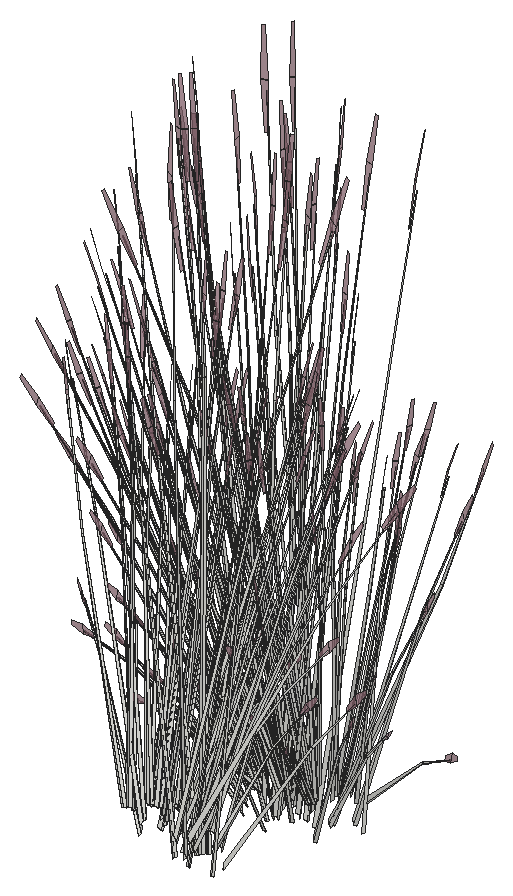
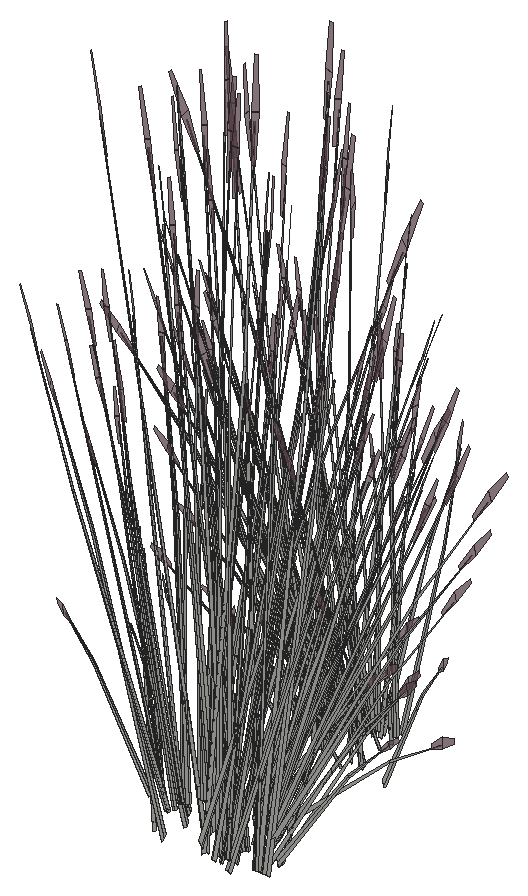
# SketchUp Ruby script. Lengths in inches.
U = 1.inch
M = Sketchup.active_model
def pt(a) = Geom::Point3d.new(a.map { |v| v * U })
def face(e, loops, mat)
  f = e.add_face(loops[0].map { |a| pt(a) })
  loops[1..].each { |l| e.add_face(l.map { |a| pt(a) }).erase! }
  f.material = f.back_material = mat if mat
  f
end
# faces: each face lists its corners as indices into pts; further lists are holes
def faces(e, pts, list, mat = nil) = list.each { |f| face(e, (f[0].is_a?(Array) ? f : [f]).map { |l| l.map { |i| pts[i] } }, mat) }
# xy, xz, yz: faces in a plane at the given z, y or x. An outline is a flat list of corners, or four numbers for a rectangle; further outlines are holes
def ring(l) = l.size == 4 ? [[l[0], l[1]], [l[2], l[1]], [l[2], l[3]], [l[0], l[3]]] : l.each_slice(2).to_a
def flat(e, list, mat, &to3) = list.each { |f| face(e, (f[0].is_a?(Array) ? f : [f]).map { |l| ring(l).map { |u, v| to3.(u, v) } }, mat) }
def xy(e, z, list, mat = nil) = flat(e, list, mat) { |x, y| [x, y, z] }
def xz(e, y, list, mat = nil) = flat(e, list, mat) { |x, z| [x, y, z] }
def yz(e, x, list, mat = nil) = flat(e, list, mat) { |y, z| [x, y, z] }
def lines(e, pts, list) = list.each { |a, b| e.add_line(pt(pts[a]), pt(pts[b])) }
# prism: a flat outline (further loops are holes) pulled along v
def prism(e, loops, v, mat = nil)
  f = face(e, loops, mat); d = Geom::Vector3d.new(v.map { |x| x * U })
  f.pushpull(f.normal.samedirection?(d) ? d.length : -d.length)
end
def box(e, o, s, mat = nil) = prism(e, [[o, [o[0] + s[0], o[1], o[2]], [o[0] + s[0], o[1] + s[1], o[2]], [o[0], o[1] + s[1], o[2]]]], [0, 0, s[2]], mat)
def at(x, y, z, deg = 0) = Geom::Transformation.translation(pt([x, y, z])) * Geom::Transformation.rotation(ORIGIN, Z_AXIS, deg.degrees)
def axes(o, x, y, z) = Geom::Transformation.new([*x, 0, *y, 0, *z, 0, *pt(o).to_a, 1])
def part(name) = M.definitions.add(name)
# library, detail: a bought-in or finely detailed component or shape, given as its bounding box
def library(name, o, s) = part(name).tap { |d| box(d.entities, o, s) }
def detail(e, o, s) = box(e.add_group.entities, o, s)
def put(e, d, t, mat = nil) = e.add_instance(d, t).tap { |i| i.material = mat if mat }
def group(e, t, mat = nil) = e.add_group.tap { |g| g.transformation = t; g.material = mat if mat }.entities
root = M.entities
M.materials.add("LightPink_Translucent").color = [144, 107, 117]
M.materials["LightPink_Translucent"].alpha = 0.75
c1 = part("blade")
p = [[2.15,0.21,22],[0,0.17,0],[0.09,0.45,0],[2.18,0.31,22],[2.29,0.31,22],[0.38,0.45,0],
  [2.48,0.24,33],[2.49,0.24,33],[2.48,0.22,33]]
faces(c1.entities,p,[[0,1,2,3],[4,5,2,3],[6,3,4,7],[8,0,3,6]])
c2 = part("seeds")
p = [[0.3,-0.1,1.38],[-0.01,-0.03,1.59],[-0.01,-0.03,0.03],[0.14,-0.07,-0.07],[0.29,-0.03,3],[0.15,0.01,3.11]]
faces(c2.entities,p,[[0,1,2,3],[1,0,4,5]],"LightPink_Translucent")
c3 = part("blade with seeds")
put(c3.entities,c1,at(0,0,0))
put(c3.entities,c2,axes([2.4,0.25,30.99],[1.5799,-0.05474,1.17369],[-0.12525,1.92788,0.29478],[-0.07173,-0.02425,1.56792]))
put(root,c3,axes([340.3,184.53,6.82],[-0.77872,0.09325,-0.35414],[-0.20563,-0.53305,0.4572],[-0.22316,0.14318,0.87481]))
put(root,c3,axes([347.67,185.27,7.03],[-0.65964,0.42992,0.48003],[-0.5689,-0.45657,0.3958],[0.30948,0.0793,0.9933]))
put(root,c3,axes([339.17,185.73,7.9375],[0.78943,0.17416,-0.06488],[-0.24284,0.53604,-0.29416],[-0.12912,0.08139,0.97024]))
put(root,c3,axes([344.77,184.74,4.35],[-0.60257,0.49041,-0.62353],[-0.74854,-0.44469,-0.16365],[-0.24146,0.12234,1.37633]))
put(root,c3,axes([345.57,185.76,7.34],[-0.13817,-0.52554,0.35414],[0.78985,-0.13877,-0.4572],[0.21215,0.1506,0.87481]))
put(root,c3,axes([345.84,185.57,4.625],[1.11998,0.21207,0.30756],[-0.2802,0.75803,-0.36492],[-0.18537,0.09487,1.64885]))
put(root,c3,axes([345.76,186.08,4.3125],[-0.83726,0.32623,-0.49651],[-0.50045,-0.58498,0],[-0.19069,0.0743,1.57504]))
put(root,c3,axes([348.54,184.15,4.3125],[0,0.65246,-0.49651],[-1.00089,0,0],[0,0.1486,1.57504]))
put(root,c3,axes([346.04,184.22,6.17],[-0.3323,-0.11241,1.71376],[0.68769,-0.4716,0.13857],[0.42861,0.21275,0.73262]))
put(root,c3,axes([346.1,182.74,6.77],[-0.77304,-0.33901,1.38283],[0.81626,-0.52782,0.59665],[0.24941,0.31809,1.33663]))
put(root,c3,axes([340.53,184.17,7.33],[0.82753,0.35977,-0.1216],[-0.47675,0.52101,-0.67495],[-0.2338,0.18111,1.02557]))
put(root,c3,axes([347.27,185.5,5.06],[-0.5037,-0.18761,1.1486],[0.6504,-0.19062,0.84392],[0.17543,0.16147,0.25299]))
put(root,c3,axes([345.5,186.04,7.33],[0.53309,-0.55848,-0.1216],[0.77201,0.32175,-0.67495],[0.26836,0.15779,1.02557]))
put(root,c3,axes([341.64,184.01,6.17],[0.22344,-0.20048,1.71376],[0.56419,0.54113,0.13857],[-0.38697,0.24643,0.73262]))
put(root,c3,axes([340.94,184.6,6.97],[0.22982,0.59576,-0.51099],[-0.87033,0.10422,-0.3958],[-0.24941,0.16002,0.97773]))
put(root,c3,axes([341.98,185.28,7.34],[0.60531,-0.34352,0.35414],[0.573,0.39225,-0.4572],[-0.08718,0.19929,0.87481]))
put(root,c3,axes([346.52,185.98,4.67],[0.55932,0.6538,0],[-0.93577,0.36461,-0.51607],[-0.21313,0.08304,1.63711]))
put(root,c3,axes([344.8,186.5,7],[0.00265,-0.07899,1.77383],[0.76665,-0.34851,-0.16761],[0.2663,0.12439,0.31391]))
put(root,c3,axes([347.41,186.2,3.79],[0.06518,-0.0942,1.76342],[0.82057,-0.27742,-0.26939],[0.24877,0.14358,0.30037]))
put(root,c3,axes([346.04,183.39,5.13],[-0.02444,-0.61432,1.41272],[1.10603,0.15924,0.59816],[-0.26159,0.33615,1.3335]))
put(root,c3,axes([346.33,184.06,4.39],[0.32803,0.59738,-0.69212],[-0.94492,0.21515,-0.18165],[0.03626,0.20229,1.52773]))
put(root,c3,axes([341.4375,185.59,7.02],[-0.73517,-0.0304,0.0643],[0.02016,-0.45906,0.50621],[-0.07693,0.17585,0.77189]))
put(root,c3,axes([339.875,186.12,3.79],[0.12,0.06519,1.76342],[0.20347,0.60397,-0.26939],[-0.26596,0.12879,0.30037]))
put(root,c3,axes([341.67,185.63,7.03],[-0.63704,-0.44518,0.48003],[0.67652,-0.38394,0.3958],[-0.11751,0.20886,0.9933]))
put(root,c3,axes([346.13,185.76,6.97],[0.88277,-0.1551,-0.51099],[0.15442,0.58737,-0.3958],[0.23711,0.16832,0.97773]))
put(root,c3,axes([343.68,185.85,7.34],[0.2697,-0.50175,0.35414],[0.78684,0.14635,-0.4572],[0.07215,0.20201,0.87481]))
put(root,c3,axes([347.35,186.35,4.96],[-0.57368,-0.02046,1.0506],[0.37886,-0.43461,0.58006],[0.22663,0.15441,0.8241]))
put(root,c3,axes([345.7,186.24,7.02],[-0.4066,0.41448,0.0643],[-0.57901,-0.24131,0.50621],[0.18719,0.13288,0.77189]))
put(root,c3,axes([344.74,187.64,7.9375],[0.61821,-0.37431,-0.06488],[0.56645,0.40995,-0.29416],[0.03988,0.11616,0.97024]))
put(root,c3,axes([345.87,186.125,7.03],[-0.88979,0.14973,0.48003],[-0.15442,-0.58737,0.3958],[0.20926,0.17311,0.9933]))
put(root,c3,axes([341.48,184.5,6.17],[0.16657,-0.22426,1.71376],[0.69879,0.4641,0.13857],[-0.31524,0.28926,0.73262]))
put(root,c3,axes([345.48,185.3,4.88],[0.01579,-0.21629,1.43002],[0.75442,-0.24159,-0.30754],[0.23289,0.25887,0.61141]))
put(root,c3,axes([343.4375,186.3,7.02],[-0.6592,0.22175,0.0643],[-0.32265,-0.40436,0.50621],[0.06366,0.17825,0.77189]))
put(root,c3,axes([341.67,185.77,6.82],[-0.60531,0.34352,-0.35414],[-0.573,-0.39225,0.4572],[-0.08718,0.19929,0.87481]))
put(root,c3,axes([339.58,185.67,7.01],[-0.02224,0.12912,1.74944],[0.63107,0.44917,-0.27667],[-0.16521,0.21241,0.14031]))
put(root,c3,axes([341.6,185.375,7.69],[0.98321,0.03233,-0.13498],[-0.02687,0.61208,-0.74919],[-0.0683,0.23574,1.13838]))
put(root,c3,axes([343.42,186.06,7.33],[0.87543,-0.30377,-0.1216],[0.4302,0.53915,-0.67495],[0.1155,0.2272,1.02557]))
put(root,c3,axes([343.67,186.26,7.36],[-0.88151,-0.17057,0.53283],[0.30143,-0.56078,0.43934],[0.05297,0.22053,1.10256]))
put(root,c3,axes([342.05,187.1,5.06],[-0.02315,-0.38796,1.1486],[0.57853,0.27671,0.84392],[-0.11378,0.18492,0.25299]))
put(root,c3,axes([343.58,186.18,3.79],[0.14478,-0.0355,1.76342],[0.8709,0.19542,-0.26939],[0.02547,0.22025,0.30037]))
put(root,c3,axes([342.27,185.61,7.3],[0.64041,0.4384,-0.5672],[-0.67652,0.38394,-0.43934],[-0.09744,0.22274,1.08528]))
put(root,c3,axes([341.57,186.26,5.12],[0.8127,-0.11554,0.06507],[0.18684,0.46549,-0.86304],[-0.05152,0.23564,0.7736]))
put(root,c3,axes([344.17,186.03,6.97],[0.87941,0.16356,-0.51099],[-0.30143,0.56078,-0.3958],[0.08064,0.22578,0.97773]))
put(root,c3,axes([344.67,184.875,6.17],[-0.2045,-0.20949,1.71376],[0.94495,-0.17636,0.13857],[0.21357,0.32887,0.73262]))
put(root,c3,axes([343.77,186.375,6.82],[-0.2697,0.50175,-0.35414],[-0.78684,-0.14635,0.4572],[0.07215,0.20201,0.87481]))
put(root,c3,axes([342.42,196.51,3.875],[0.2045,0.20949,1.71376],[-0.94495,0.17636,0.13857],[-0.21357,-0.32887,0.73262]))
put(root,c3,axes([342.07,185.41,7.63],[-0.02328,0.60353,-0.7886],[-0.98022,-0.04053,0.09517],[-0.10344,0.25568,1.11556]))
put(root,c3,axes([339.51,186.99,7],[0.10149,-0.03939,1.77383],[0.83886,0.26202,-0.16761],[-0.01971,0.21816,0.31391]))
put(root,c3,axes([343.98,195.12,4.72],[-0.13683,-0.09148,1.74944],[-0.91315,0.058,-0.27667],[-0.14574,-0.2188,0.14031]))
put(root,c3,axes([343,184.98,6.17],[-0.0219,-0.25042,1.71376],[0.94901,0.16613,0.13857],[-0.0587,0.35688,0.73262]))
put(root,c3,axes([346.1,196.2,2.59],[-0.25429,0.13207,1.43002],[-0.76157,-0.23115,-0.30754],[0.14117,-0.28747,0.61141]))
put(root,c3,axes([344.94,196.66,4.98],[-0.42698,-0.53052,-0.71045],[0.87893,-0.29566,0.08574],[-0.09984,-0.25633,1.00501]))
put(root,c3,axes([342.16,195.95,2.59],[-0.05417,0.21344,1.43002],[-0.79196,0.17867,-0.30754],[-0.18512,-0.27588,0.61141]))
put(root,c3,axes([343.85,185.92,7.27],[0.42698,0.53052,-0.71045],[-0.87893,0.29566,0.08574],[0.09984,0.25633,1.00501]))
put(root,c3,axes([344.2,195.49,1.49],[-0.15005,0.02351,1.76342],[-0.82981,-0.26461,-0.26939],[0.01392,-0.22072,0.30037]))
put(root,c3,axes([341.38,186.76,4.88],[0.28231,-0.10293,1.43002],[0.69701,0.31035,-0.30754],[-0.20746,0.26854,0.61141]))
put(root,c3,axes([343.21,187.26,7.01],[0.1134,0.10507,1.74944],[0.91515,0.04128,-0.27667],[0.09203,0.23172,0.14031]))
put(root,c3,axes([346.72,197.18,4.98],[0.02328,-0.60353,-0.71045],[0.98022,0.04053,0.08574],[0.10344,-0.25568,1.00501]))
put(root,c3,axes([348.09,196.24,4.72],[-0.00864,-0.12985,1.74944],[-0.72937,-0.3753,-0.27667],[0.11277,-0.2275,0.14031]))
put(root,c3,axes([345.02,196.21,4.53],[0.2697,-0.50175,-0.35414],[0.78684,0.14635,0.4572],[-0.07215,-0.20201,0.87481]))
put(root,c3,axes([345.62,196.875,3.875],[-0.16657,0.22426,1.71376],[-0.69879,-0.4641,0.13857],[0.31524,-0.28926,0.73262]))
put(root,c3,axes([347.89,195.77,4.71],[-0.09085,0.04984,1.77383],[-0.89014,-0.16814,-0.16761],[-0.03222,-0.21748,0.31391]))
put(root,c3,axes([344.62,196.56,4.68],[-0.87941,-0.16356,-0.51099],[0.30143,-0.56078,-0.3958],[-0.08064,-0.22578,0.97773]))
put(root,c3,axes([345.16,195.15,2.77],[0.11476,0.38047,1.1486],[-0.63664,-0.21072,0.84392],[0.06851,-0.19481,0.25299]))
put(root,c3,axes([346.52,196.98,4.68],[-0.64041,-0.4384,-0.51099],[0.67652,-0.38394,-0.3958],[0.09744,-0.22274,0.97773]))
put(root,c3,axes([341.74,186.26,5.66],[0.01966,-0.33682,1.54345],[0.88405,0.17791,0.21329],[-0.0766,0.35897,0.72882]))
put(root,c3,axes([343.05,194.82,4.71],[-0.01669,0.07821,1.77383],[-0.82314,0.28383,-0.16761],[-0.24223,-0.14508,0.31391]))
put(root,c3,axes([342.87,196.21,5.09],[0.99656,-0.1677,0.53763],[0.17295,0.65785,0.4433],[-0.23438,-0.19388,1.11249]))
put(root,c3,axes([345.12,196.33,4.73],[0.88151,0.17057,0.48003],[-0.30143,0.56078,0.3958],[-0.05297,-0.22053,0.9933]))
put(root,c3,axes([345.37,196.53,5.03],[-0.87543,0.30377,-0.1216],[-0.4302,-0.53915,-0.67495],[-0.1155,-0.2272,1.02557]))
put(root,c3,axes([347.19,197.21,5.03],[-0.98321,-0.03233,-0.1216],[0.02687,-0.61208,-0.67495],[0.0683,-0.23574,1.02557]))
put(root,c3,axes([347.12,196.82,4.53],[0.60531,-0.34352,-0.35414],[0.573,0.39225,0.4572],[0.08718,-0.19929,0.87481]))
put(root,c3,axes([341.89,195.61,2.77],[0.46666,0.22709,1.1486],[-0.67962,0.13651,0.84392],[-0.14541,-0.17452,0.25299]))
put(root,c3,axes([345.35,196.29,4.73],[0.6592,-0.22175,0.0643],[0.32265,0.40436,0.50621],[-0.06366,-0.17825,0.77189]))
put(root,c3,axes([343.02,196.8125,4.98],[-0.76283,-0.31537,-0.71045],[0.54213,-0.55263,0.08574],[-0.27638,-0.1883,1.00501]))
put(root,c3,axes([342.75,196.4,4.53],[-0.13817,-0.52554,-0.35414],[0.78985,-0.13877,0.4572],[-0.21215,-0.1506,0.87481]))
put(root,c3,axes([343.09,196.35,4.73],[0.4066,-0.41448,0.0643],[0.57901,0.24131,0.50621],[-0.18719,-0.13288,0.77189]))
put(root,c3,axes([341.52,196.29,1.49],[-0.08666,0.08595,1.76342],[-0.87574,0.18531,-0.26939],[-0.21156,-0.16858,0.30037]))
put(root,c3,axes([342.97,198.65,2.1],[-0.36739,-0.66907,-0.69835],[1.05831,-0.24096,-0.18329],[-0.04061,-0.22656,1.54149]))
put(root,c3,axes([341.05,197.16,3.875],[0.3323,0.11241,1.71376],[-0.68769,0.4716,0.13857],[-0.42861,-0.21275,0.73262]))
put(root,c3,axes([347.88,196.61,1.49],[-0.1339,-0.0514,1.76342],[-0.34394,-0.57425,-0.26939],[0.23202,-0.15583,0.30037]))
put(root,c3,axes([345.11,196.74,5.05],[-0.2697,0.50175,0.35414],[-0.78684,-0.14635,-0.4572],[-0.07215,-0.20201,0.87481]))
put(root,c3,axes([342.66,196.83,4.68],[-0.88277,0.1551,-0.51099],[-0.15442,-0.58737,-0.3958],[-0.23711,-0.16832,0.97773]))
put(root,c3,axes([347.12,196.95,4.73],[0.63704,0.44518,0.48003],[-0.67652,0.38394,0.3958],[0.11751,-0.20886,0.9933]))
put(root,c3,axes([343.28,196.3,5.43],[-0.59706,0.6255,-0.13619],[-0.86465,-0.36036,-0.75594],[-0.30056,-0.17672,1.14864]))
put(root,c3,axes([347.36,196.99,4.73],[0.73517,0.0304,0.0643],[-0.02016,0.45906,0.50621],[0.07693,-0.17585,0.77189]))
put(root,c3,axes([346.81,197.31,5.05],[-0.60531,0.34352,0.35414],[-0.573,-0.39225,-0.4572],[0.08718,-0.19929,0.87481]))
put(root,c3,axes([347.875,198.23,4.98],[0.4673,-0.51481,-0.71045],[0.81887,0.36587,0.08574],[0.27902,-0.18652,1.00501]))
put(root,c3,axes([342.82,196.73,2.375],[-0.55932,-0.6538,0],[0.93577,-0.36461,-0.51607],[0.21313,-0.08304,1.63711]))
put(root,c3,axes([347.85,197.99,4.68],[-0.22982,-0.59576,-0.51099],[0.87033,-0.10422,-0.3958],[0.24941,-0.16002,0.97773]))
put(root,c3,axes([344.05,195.94,2.13],[-0.61821,0.37431,-0.03893],[-0.56645,-0.40995,-0.17649],[-0.03988,-0.11616,0.58215]))
put(root,c3,axes([340.99,196.125,4.72],[-0.19249,-0.00461,1.74944],[-0.61281,0.46055,-0.27667],[-0.32697,-0.0941,0.14031]))
put(root,c3,axes([348.26,198.42,5.03],[-0.82753,-0.35977,-0.1216],[0.47675,-0.52101,-0.67495],[0.2338,-0.18111,1.02557]))
put(root,c3,axes([344.84,200.38,3.33],[0.77308,0.2631,1.51261],[-0.75736,0.56681,0.59816],[-0.33924,-0.33594,1.26806]))
put(root,c3,axes([343.22,196.82,5.05],[0.13817,0.52554,0.35414],[-0.78985,0.13877,-0.4572],[-0.21215,-0.1506,0.87481]))
put(root,c3,axes([340.8,198.5625,2.02],[0,-0.65246,-0.49651],[1.00089,0,0],[0,-0.1486,1.57504]))
put(root,c3,axes([343.58,196.63,2.02],[0.83726,-0.32623,-0.49651],[0.50045,0.58498,0],[0.19069,-0.0743,1.57504]))
put(root,c3,axes([348.55,197.76,2.59],[-0.31959,-0.01933,1.43002],[-0.32741,-0.51843,-0.30754],[0.39262,-0.14666,0.61141]))
put(root,c3,axes([340.85,197.17,5.09],[0.7388,-0.48151,0.53763],[0.63717,0.51135,0.4433],[-0.34662,-0.08882,1.11249]))
put(root,c3,axes([350.3,198.26,4.71],[-0.11685,-0.00496,1.77383],[-0.48522,-0.53096,-0.16761],[0.19486,-0.17458,0.31391]))
put(root,c3,axes([344.57,197.97,2.06],[0.60257,-0.49041,-0.62353],[0.74854,0.44469,-0.16365],[0.24146,-0.12234,1.37633]))
put(root,c3,axes([348.92,196.8,2.77],[-0.29798,0.33213,1.1486],[-0.25612,-0.44624,0.84392],[0.24611,-0.11182,0.25299]))
put(root,c3,axes([348.49,198.05,4.53],[0.77872,-0.09325,-0.35414],[0.20563,0.53305,0.4572],[0.22316,-0.14318,0.87481]))
put(root,c3,axes([341.19,197.16,4.73],[0.04505,-0.49615,0.0643],[0.68022,0.0136,0.50621],[-0.26056,-0.05192,0.77189]))
put(root,c3,axes([343.53,198.83,2.21],[0.43405,-0.58792,-0.44739],[0.90188,0.28295,0.21531],[0,-0.13553,1.43643]))
put(root,c3,axes([340.92,197.32,4.53],[-0.50902,-0.40851,-0.35414],[0.58122,-0.38671,0.4572],[-0.29531,-0.05884,0.87481]))
put(root,c3,axes([343.92,198.54,2.67],[-0.10425,-0.7445,-0.29095],[1.08575,-0.04502,-0.50002],[0.19119,-0.09917,1.59708]))
put(root,c3,axes([341.23,198.58,2.03],[0.62448,-0.40708,-0.30978],[0.62448,0.40708,0.30978],[0,-0.13112,1.38974]))
put(root,c3,axes([340.98,196.625,2.13],[-0.25807,0.53277,-0.03893],[-0.79428,-0.16389,-0.17649],[-0.1206,-0.08714,0.58215]))
put(root,c3,axes([347.86,198.37,5.05],[-0.77872,0.09325,0.35414],[-0.20563,-0.53305,-0.4572],[0.22316,-0.14318,0.87481]))
put(root,c3,axes([343.42,199.32,2.67],[-1.00749,-0.31132,-0.29095],[0.48511,-0.65709,-0.50002],[-0.03166,-0.16133,1.59708]))
put(root,c3,axes([340.55,199.06,2.375],[-1.11865,0,0],[0,-0.72922,-0.51607],[0,-0.16609,1.63711]))
put(root,c3,axes([340.74,197.75,2.59],[0.17466,0.18165,1.43002],[-0.40248,0.49377,-0.30754],[-0.41327,-0.11802,0.61141]))
put(root,c3,axes([343.78,196.89,2.03],[0.83462,0.16144,-0.30978],[-0.21015,0.56852,0.30978],[0.16826,-0.06556,1.38974]))
put(root,c3,axes([341.46,197.59,4.98],[-0.89428,-0.01571,-0.71045],[0.06006,-0.66153,0.08574],[-0.37886,-0.06981,1.00501]))
put(root,c3,axes([348.5625,198.28,4.73],[0.61415,0.2744,0.0643],[-0.35756,0.39076,0.50621],[0.1969,-0.12633,0.77189]))
put(root,c3,axes([348.39,198.17,4.73],[0.22187,0.60049,0.48003],[-0.87033,0.10422,0.3958],[0.25651,-0.14123,0.9933]))
put(root,c3,axes([350.74,198.89,4.72],[0.12414,-0.09938,1.74944],[-0.15889,-0.60963,-0.27667],[0.31148,-0.11559,0.14031]))
put(root,c3,axes([341.42,198.86,2.33],[-0.83213,0.54855,0.30756],[-0.83263,-0.54278,-0.36492],[-0.02906,-0.15578,1.64885]))
put(root,c3,axes([340.25,196.51,4.71],[0.06632,0.06511,1.77383],[-0.31973,0.58531,-0.16761],[-0.32381,0.00424,0.31391]))
put(root,c3,axes([344.0625,199.12,2.43],[1.00799,0.31623,0.24065],[-0.48511,0.65709,0.50002],[0,-0.15147,1.60543]))
put(root,c3,axes([343.67,200.01,2.4375],[0.23711,-0.77313,-0.23429],[1.12425,0.13477,0.51271],[-0.19645,-0.10677,1.5644]))
put(root,c3,axes([341.17,197.73,4.68],[-0.6496,0.4322,-0.51099],[-0.5689,-0.45657,-0.3958],[-0.33005,-0.06576,0.97773]))
put(root,c3,axes([341.65,197.53,5.05],[0.50902,0.40851,0.35414],[-0.58122,0.38671,-0.4572],[-0.29531,-0.05884,0.87481]))
put(root,c3,axes([339.7,198.3,2.77],[0.57115,-0.04669,1.1486],[-0.36229,0.41137,0.84392],[-0.28224,-0.06171,0.25299]))
put(root,c3,axes([343.74,198.68,2.72],[-0.97146,0.04028,0.44739],[-0.08785,-0.66859,-0.21531],[0.17391,-0.06776,1.43643]))
put(root,c3,axes([341.51,197.27,5.03],[-0.0479,0.66354,-0.1216],[-0.90696,-0.01814,-0.67495],[-0.3493,-0.04609,1.02557]))
put(root,c3,axes([341.23,199.17,2.48],[0,0.65246,0.49651],[-1.00089,0,0],[0,-0.1486,1.57504]))
put(root,c3,axes([348.29,199.82,5.03],[-0.45012,-0.59081,-0.1216],[0.79888,-0.29033,-0.67495],[0.33665,-0.07795,1.02557]))
put(root,c3,axes([348.26,199.3125,4.68],[0.24236,-0.59349,-0.51099],[0.83094,0.20343,-0.3958],[0.33455,-0.05442,0.97773]))
put(root,c3,axes([346.94,196.9,2.375],[0.55932,-0.6538,0],[0.93577,0.36461,-0.51607],[0.21313,0.08304,1.63711]))
put(root,c3,axes([340.35,198.1875,3.875],[0.37107,-0.01478,1.71376],[-0.24616,0.64047,0.13857],[-0.5288,-0.03961,0.73262]))
put(root,c3,axes([343.59,199.69,2.21],[-0.53742,-0.54764,-0.44739],[0.81403,-0.38564,0.21531],[-0.17391,-0.06776,1.43643]))
put(root,c3,axes([343.7,198.92,2.36],[0.38895,0.72959,0.45755],[-1.11135,0.2537,0.17955],[0.01358,-0.13406,1.58856]))
put(root,c3,axes([349.14,199.48,1.98],[-0.57619,0.0783,1.41583],[-0.09171,-0.62326,0.08104],[0.40356,-0.09434,0.80566]))
put(root,c3,axes([350.19,198.93,2.26],[-0.55463,-0.41721,-0.06488],[0.60744,-0.38228,-0.29416],[0.17212,-0.02691,0.97024]))
put(root,c3,axes([343.51,199.49,2.72],[-0.43405,0.58792,0.44739],[-0.90188,-0.28295,-0.21531],[0,-0.13553,1.43643]))
put(root,c3,axes([345.1,198.98,2.21],[0,-0.75495,0],[1.11865,0,0],[0,0,1.79456]))
put(root,c3,axes([346.46,197.24,2.48],[-0.83726,-0.32623,0.49651],[0.50045,-0.58498,0],[0.19069,0.0743,1.57504]))
put(root,c3,axes([348.1,199.53,4.98],[0.78611,-0.28816,-0.71045],[0.4381,0.59317,0.08574],[0.37982,-0.06738,1.00501]))
put(root,c3,axes([343.11,199.9,2.06],[-0.9306,-0.10697,-0.62353],[0.19638,-0.65984,-0.16365],[-0.27771,-0.07995,1.37633]))
put(root,c3,axes([344.57,198.51,2.36],[-0.74176,0.59212,0.45755],[-0.88124,-0.52269,0.17955],[0.17882,-0.05909,1.58856]))
put(root,c3,axes([345.38,199.57,2.3],[-0.83213,-0.56158,-0.06131],[0.83263,-0.56193,0],[-0.02906,-0.01961,1.75571]))
put(root,c3,axes([343.29,197.53,2.47],[-0.25843,0.64844,0.17642],[-0.9457,-0.1835,0.35086],[0.16336,-0.00316,1.60407]))
put(root,c3,axes([347.98,199.64,5.05],[-0.74348,-0.18202,0.35414],[0.21685,-0.53102,-0.4572],[0.29933,-0.04869,0.87481]))
